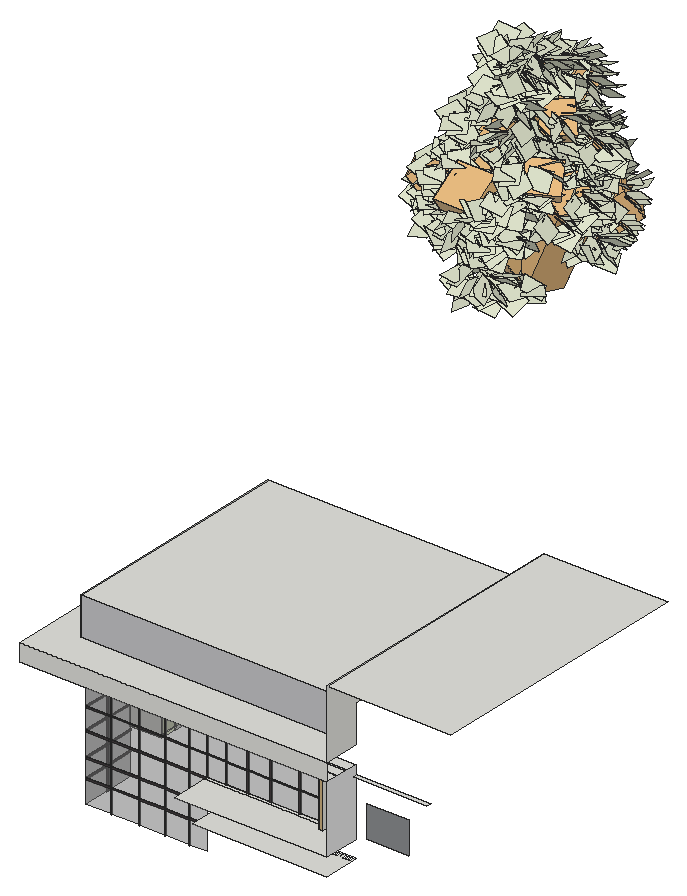
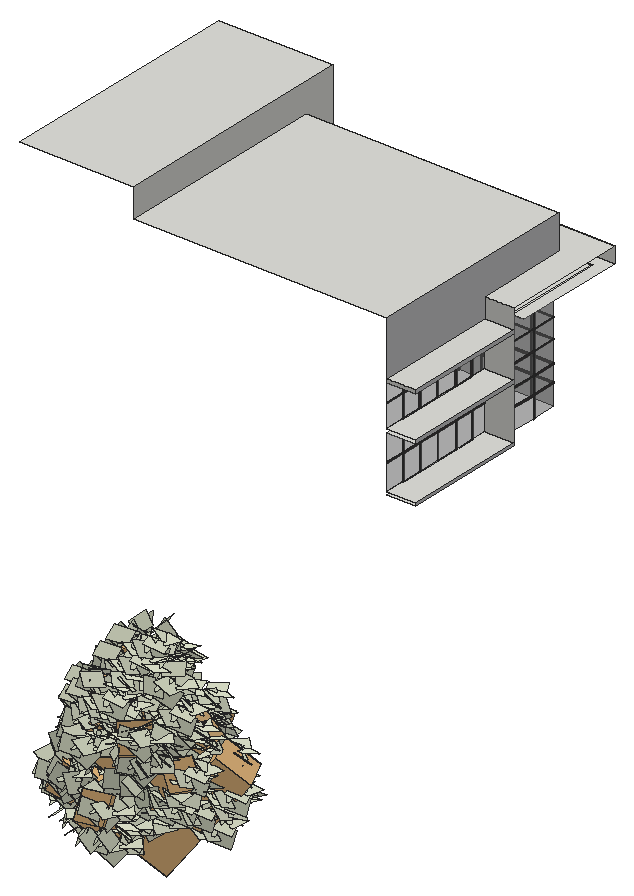
# SketchUp Ruby script. Lengths in inches.
U = 1.inch
M = Sketchup.active_model
def pt(a) = Geom::Point3d.new(a.map { |v| v * U })
def face(e, loops, mat)
  f = e.add_face(loops[0].map { |a| pt(a) })
  loops[1..].each { |l| e.add_face(l.map { |a| pt(a) }).erase! }
  f.material = f.back_material = mat if mat
  f
end
# faces: each face lists its corners as indices into pts; further lists are holes
def faces(e, pts, list, mat = nil) = list.each { |f| face(e, (f[0].is_a?(Array) ? f : [f]).map { |l| l.map { |i| pts[i] } }, mat) }
# xy, xz, yz: faces in a plane at the given z, y or x. An outline is a flat list of corners, or four numbers for a rectangle; further outlines are holes
def ring(l) = l.size == 4 ? [[l[0], l[1]], [l[2], l[1]], [l[2], l[3]], [l[0], l[3]]] : l.each_slice(2).to_a
def flat(e, list, mat, &to3) = list.each { |f| face(e, (f[0].is_a?(Array) ? f : [f]).map { |l| ring(l).map { |u, v| to3.(u, v) } }, mat) }
def xy(e, z, list, mat = nil) = flat(e, list, mat) { |x, y| [x, y, z] }
def xz(e, y, list, mat = nil) = flat(e, list, mat) { |x, z| [x, y, z] }
def yz(e, x, list, mat = nil) = flat(e, list, mat) { |y, z| [x, y, z] }
def lines(e, pts, list) = list.each { |a, b| e.add_line(pt(pts[a]), pt(pts[b])) }
# prism: a flat outline (further loops are holes) pulled along v
def prism(e, loops, v, mat = nil)
  f = face(e, loops, mat); d = Geom::Vector3d.new(v.map { |x| x * U })
  f.pushpull(f.normal.samedirection?(d) ? d.length : -d.length)
end
def box(e, o, s, mat = nil) = prism(e, [[o, [o[0] + s[0], o[1], o[2]], [o[0] + s[0], o[1] + s[1], o[2]], [o[0], o[1] + s[1], o[2]]]], [0, 0, s[2]], mat)
def at(x, y, z, deg = 0) = Geom::Transformation.translation(pt([x, y, z])) * Geom::Transformation.rotation(ORIGIN, Z_AXIS, deg.degrees)
def axes(o, x, y, z) = Geom::Transformation.new([*x, 0, *y, 0, *z, 0, *pt(o).to_a, 1])
def part(name) = M.definitions.add(name)
# library, detail: a bought-in or finely detailed component or shape, given as its bounding box
def library(name, o, s) = part(name).tap { |d| box(d.entities, o, s) }
def detail(e, o, s) = box(e.add_group.entities, o, s)
def put(e, d, t, mat = nil) = e.add_instance(d, t).tap { |i| i.material = mat if mat }
def group(e, t, mat = nil) = e.add_group.tap { |g| g.transformation = t; g.material = mat if mat }.entities
root = M.entities
M.materials.add("Celtis_australis_s cópia1").color = [224, 229, 205]
M.materials.add("Screenshot").color = [140, 142, 145]
M.materials.add("[Asphalt New]").color = [67, 60, 62]
M.materials.add("[Polished Concrete New]").color = [200, 200, 203]
M.materials.add("[Polished Concrete Old]").color = [229, 229, 229]
M.materials.add("[Translucent Glass Gray]").color = [128, 128, 128]
M.materials["[Translucent Glass Gray]"].alpha = 0.5
M.materials.add("[Wood Floor Light]").color = [204, 176, 127]
M.materials.add("bark_cherry").color = [99, 76, 62]
c1 = part("branch2\#1")
p = [[13.74,0.36,0.5],[11.5,11.3125,10.98],[14.125,0.95,0],[14.97,0.95,0.19],[12.12,10.6875,11.67],[15.1,0.36,0.82],
  [11.05,10.4375,11.49],[14.34,0,1.01],[6.08,18.54,23.51],[6.83,18.32,23.89],[6.09,17.93,24.13],[3.27,29.37,34],
  [3.27,29.68,33.56],[3.73,29.59,33.82],[0,43.16,40.74],[0,43.16,40.75],[0.01,43.16,40.75],[5.59,23.2,32.77],
  [4.65,30.48,39.08],[1.92,39.79,43.02],[5.09,28.47,41.41]]
faces(c1.entities,p,[[0,1,2],[2,1,3],[3,4,5],[3,1,4],[6,0,7],[0,6,1],[5,6,7],[6,5,4],
  [6,8,1],[1,9,4],[9,1,8],[8,6,10],[4,10,6],[10,4,9],[10,11,8],[8,12,9],
  [12,8,11],[10,9,11],[13,11,9],[13,9,12],[14,12,11,15],[12,14,16,13],[13,16,15,11]],"bark_cherry")
lines(c1.entities,p,[[17,18],[11,19],[20,17],[17,10]])
c2 = library("branch1\#2",[0,0,0],[33.4,33.29,108.01])
c3 = part("leaf1\#1")
p = [[1.6,6.78,0.04],[-9.34,-4.04,0.02],[2.67,-16.2,2.05],[13.62,-5.38,2.07]]
faces(c3.entities,p,[[0,1,2,3]],"Celtis_australis_s cópia1")
c4 = part("leaf_group1\#1")
put(c4.entities,c3,axes([-0.06,3.68,7.3125],[0.53029,-0.80282,-0.27253],[0.82812,0.42159,0.36943],[-0.18168,-0.42159,0.8884]))
put(c4.entities,c3,axes([6.4375,-3.58,5.23],[1,0,0],[0,0.98927,0.14608],[0,-0.14608,0.98927]))
put(c4.entities,c3,axes([-0.99,3.68,1.22],[0.57591,-0.80282,0.15431],[0.36532,0.42159,0.82994],[-0.73135,-0.42159,0.53609]))
put(c4.entities,c3,axes([18.71,8.59,4.39],[0.33053,0.77491,0.53877],[-0.79988,-0.073,0.5957],[0.50094,-0.62785,0.5957]))
put(c4.entities,c3,axes([13.16,0.76,0.89],[0.89618,0.3501,0.27256],[-0.44248,0.65988,0.60727],[0.03275,-0.66482,0.74628]))
put(c4.entities,c3,axes([4.53,7.98,7.3125],[-0.1927,0.94265,-0.27253],[0.88368,0.28746,0.36943],[-0.42658,0.16964,0.8884]))
put(c4.entities,c3,axes([12.46,21.28,7.16],[0.85019,0.38493,0.35918],[0.30538,-0.91629,0.25914],[-0.42887,0.11063,0.89657]))
put(c4.entities,c3,axes([6.53,15.18,2.59],[0.70711,0.70711,0],[0.5,-0.5,0.70711],[-0.5,0.5,0.70711]))
put(c4.entities,c3,axes([-3.17,8.15,3.46],[-0.03719,0.74973,0.66069],[0.94096,-0.19634,0.27576],[-0.33647,-0.63194,0.69817]))
put(c4.entities,c3,axes([23.03,17.79,4.39],[0.78166,-0.31422,0.53877],[-0.61722,-0.51398,0.5957],[-0.08973,0.79818,0.5957]))
put(c4.entities,c3,axes([14.78,21.52,3.21],[0.67246,-0.04394,0.73882],[-0.28657,-0.93583,0.20517],[-0.6824,0.3497,0.64191]))
put(c4.entities,c3,axes([10.37,-1.8125,9],[0.99279,-0.06448,-0.101],[0.11527,0.74421,0.65792],[0.03275,-0.66482,0.74628]))
put(c4.entities,c3,axes([1.45,16.1875,2.9375],[-0.2106,-0.86579,-0.45394],[0.96054,-0.26957,0.06852],[-0.18168,-0.42159,0.8884]))
c5 = part("branch3")
p = [[6.085,7.082,2.644],[4.083,0.001,0],[4.08,0.002,0.001],[5.841,7.141,2.739],[4.083,0,0.004],[6.032,7.035,2.901],
  [8.234,14.378,3.666],[10.055,21.673,1.937],[8.611,14.241,3.496],[10.247,21.661,2.456],[9.737,21.9,2.346],[9.715,21.803,2.365],
  [12.357,28.999,2.225],[12.894,28.763,2.608],[12.761,28.844,2.204],[10.064,22.087,2.083],[10.362,21.9,2.346],[5.434,16.028,3.111],
  [10.04,22.14,2.516],[12.239,29.014,2.642],[8.553,14.232,3.928],[5.628,15.927,3.273],[5.444,16.098,3.367],[12.571,28.869,2.879],
  [0.628,10.534,6.01],[0.625,10.536,6.008],[0.625,10.537,6.012],[6.135,9.846,4.735],[0.003,10.534,6.01],[0,10.537,6.012],
  [1.761,10.232,4.093],[4.16,5.476,4.049],[3.718,5.459,5.543],[3.205,0.783,1.919]]
faces(c5.entities,p,[[0,1,2,3],[3,2,4,5],[1,0,5,4],[6,7,8],[9,8,7],[7,6,10,11],[12,7,11],[13,7,14],
  [14,7,12],[13,9,7],[15,16,17],[15,17,18],[12,11,19],[20,10,6],[10,20,9,11],[21,17,16],
  [21,16,22],[18,22,16],[9,19,11],[8,9,20],[22,18,17],[9,13,23],[19,9,23],[0,8,5],
  [3,6,0],[8,0,6],[3,5,6],[20,5,8],[20,6,5],[21,24,25,17],[26,22,17,25],[22,26,24,21]],"bark_cherry")
lines(c5.entities,p,[[27,20],[28,29],[17,30],[27,31],[32,27],[5,33]])
c6 = part("branch1\#1")
p = [[23.875,19.65,51.47],[23.47,20.4,51.62],[21.1,21.64,19.5],[21.93,21.1875,19.92],[21.95,22.18,19.69],[26.48,9.62,42.86],
  [30.79,16.22,49.68],[31.01,4.77,55.38],[31.01,0,68.57],[9.91,24.21,59.69],[9.92,24.21,59.7],[24,20.54,51.64],
  [12.85,4.92,53.79],[26.1,8.92,42.74],[31.84,25.13,88.91],[31.84,25.13,106.45],[30.18,33.29,93.95],[30.18,25.42,69.53],
  [0,6.37,81.52],[11.1,10.75,77.87]]
lines(c6.entities,p,[[0,1],[2,3],[3,4],[5,6],[7,8],[9,10],[1,11],[11,0],[12,13],[4,2],[14,15],[16,17],
  [18,19]])
detail(c6.entities,[5.26,2.24,0],[28.14,24.14,108.01])
xy(root,56.77,[[542.91,273.58,570.41,390.8]])
xy(root,59.17,[[542.91,273.58,570.41,390.8]])
xy(root,86.125,[[694.73,152.69,694.73,184.77,755.09,184.77,755.09,179.27,756.79,179.27,756.79,184.77,757.59,184.77,757.59,179.27,759.29,179.27,759.29,184.77,760.09,184.77,760.09,179.27,761.79,179.27,761.79,184.77,762.59,184.77,762.59,179.27,764.29,179.27,764.29,184.77,765.09,184.77,765.09,179.27,766.79,179.27,766.79,184.77,767.59,184.77,767.59,179.27,769.29,179.27,769.29,184.77,770.09,184.77,770.09,179.27,771.79,179.27,771.79,184.77,772.59,184.77,772.59,179.27,774.29,179.27,774.29,184.77,775.09,184.77,775.09,179.27,776.79,179.27,776.79,184.77,777.59,184.77,777.59,179.27,779.29,179.27,779.29,184.77,780.09,184.77,780.09,179.27,781.79,179.27,781.79,184.77,782.59,184.77,782.59,179.27,784.29,179.27,784.29,184.77,785.09,184.77,785.09,179.27,786.79,179.27,786.79,184.77,787.59,184.77,787.59,179.27,789.29,179.27,789.29,184.77,790.09,184.77,790.09,179.27,791.79,179.27,791.79,184.77,792.59,184.77,792.59,179.27,794.29,179.27,794.29,184.77,795.47,184.77,795.47,179.27,797.16,179.27,797.16,184.77,798.34,184.77,798.34,179.27,800.04,179.27,800.04,184.77,801.22,184.77,801.22,179.27,802.91,179.27,802.91,184.77,804.09,184.77,804.09,179.27,805.79,179.27,805.79,184.77,806.97,184.77,806.97,179.27,808.66,179.27,808.66,184.77,809.84,184.77,809.84,179.27,811.54,179.27,811.54,184.77,812.47,184.77,812.47,152.69]])
xy(root,101.125,[[679.09,152.69,812.47,152.69,812.47,184.77,786.97,184.77,786.97,179.89,783.34,179.89,783.34,185.64,679.09,185.64],[679.09,185.64,783.34,188.52]])
xy(root,110.22,[[542.91,273.58,570.41,390.8]])
xy(root,113.5,[[542.91,273.58,570.41,390.8]])
xy(root,143.35,[[565.41,179.89,565.41,237.58,570.41,237.58,570.41,185.64,783.34,185.64,783.34,179.89],[570.41,185.64,570.41,188.45,572.41,185.64],[572.41,185.64,570.41,188.45,570.41,237.58,572.41,237.58,572.41,188.52,783.34,188.52,783.34,185.64]])
xy(root,146.5,[[565.41,179.89,783.34,179.89,783.34,184.77,570.41,184.77,570.41,241.02,565.41,241.02],[783.34,179.89,786.97,184.77]])
xy(root,152.71,[[542.91,273.58,570.41,390.8]])
xy(root,156.52,[[542.91,273.58,570.41,390.8]])
xy(root,160.15,[[542.91,152.69,542.91,261.08,554.03,261.08,554.03,163.32,812.47,163.32,812.47,152.69],[554.03,163.32,554.03,261.08,555.09,261.08,555.09,164.69,812.47,164.69,812.47,163.32],[555.09,164.69,555.09,261.08,559.28,261.08,559.28,173.1,812.47,173.1,812.47,164.69],[559.28,173.1,559.28,261.08,560.36,261.08,560.36,174.73,812.47,174.73,812.47,173.1],[560.36,174.73,560.36,261.08,570.41,261.08,570.41,184.77,812.47,184.77,812.47,174.73]])
xy(root,175.33,[[839.12,148.44,903.81,152.69]])
xy(root,175.35,[[542.91,152.69,812.47,152.69,812.47,184.77,570.41,184.77,570.41,273.58,542.91,273.58]])
xy(root,208.1875,[[570.41,184.77,812.47,390.8]])
xy(root,235.625,[[812.47,152.69,921.28,390.8]])
xz(root,148.44,[[850.82,130.92,887.85,158.83]],"Screenshot")
xz(root,152.69,[[542.91,160.15,812.47,175.35]])
xz(root,179.89,[[783.34,101.125,786.97,146.5],[565.41,143.35,783.34,146.5]],"[Wood Floor Light]")
xz(root,184.77,[[786.97,101.125,812.47,101.125,812.47,160.15,570.41,160.15,570.41,146.5,786.97,146.5]])
xz(root,184.77,[[570.41,175.35,812.47,208.1875]],"[Polished Concrete New]")
xz(root,188.52,[[593.95,42.44,594.71,62.36],[618.47,42.44,619.6,62.36],[641.13,42.44,642.0625,62.36],[662.45,42.44,663.59,62.36],[572.41,62.36,593.95,63.78],
  [593.95,62.36,594.71,63.78],[594.71,62.36,618.47,63.78],[618.47,62.36,619.6,63.78],[619.6,62.36,641.13,63.78],[641.13,62.36,642.0625,63.78],
  [642.0625,62.36,662.45,63.78],[662.45,62.36,663.59,63.78],[663.59,62.36,679.09,63.78],[593.95,63.78,594.71,78.79],[618.47,63.78,619.6,78.79],
  [641.13,63.78,642.0625,78.79],[662.45,63.78,663.59,78.79],[572.41,78.79,593.95,80.28],[593.95,78.79,594.71,80.28],[594.71,78.79,606.59,80.28],
  [606.59,78.79,618.47,80.28],[618.47,78.79,619.6,80.28],[619.6,78.79,641.13,80.28],[641.13,78.79,642.0625,80.28],[642.0625,78.79,662.45,80.28],
  [662.45,78.79,663.59,80.28],[663.59,78.79,679.09,80.28],[593.95,80.28,594.71,99.76],[618.47,80.28,619.6,99.76],[641.13,80.28,642.0625,99.76],
  [662.45,80.28,663.59,99.76],[572.41,99.76,593.95,101.125],[593.95,99.76,594.71,101.125],[594.71,99.76,618.47,101.125],[618.47,99.76,619.6,101.125],
  [619.6,99.76,641.13,101.125],[641.13,99.76,642.0625,101.125],[642.0625,99.76,662.45,101.125],[662.45,99.76,663.59,101.125],[663.59,99.76,679.09,101.125],
  [593.95,101.125,594.71,119.02],[618.47,101.125,619.6,119.02],[641.13,101.125,642.0625,119.02],[662.45,101.125,663.59,119.02],[678.43,101.125,679.09,119.02],
  [695.1,101.125,696.03,119.02],[713.93,101.125,715.23,119.02],[734.02,101.125,735.26,119.02],[759.3,101.125,760.48,119.02],[572.41,119.02,593.95,119.9],
  [593.95,119.02,594.71,119.9],[594.71,119.02,618.47,119.9],[618.47,119.02,619.6,119.9],[619.6,119.02,641.13,119.9],[641.13,119.02,642.0625,119.9],
  [642.0625,119.02,662.45,119.9],[662.45,119.02,663.59,119.9],[663.59,119.02,678.43,119.9],[678.43,119.02,679.09,119.9],[679.09,119.02,695.1,119.9],
  [695.1,119.02,696.03,119.9],[696.03,119.02,713.93,119.9],[713.93,119.02,715.23,119.9],[715.23,119.02,734.02,119.9],[734.02,119.02,735.26,119.9],
  [735.26,119.02,759.3,119.9],[759.3,119.02,760.48,119.9],[760.48,119.02,783.34,119.9],[593.95,119.9,594.71,143.35],[618.47,119.9,619.6,143.35],
  [641.13,119.9,642.0625,143.35],[662.45,119.9,663.59,143.35],[678.43,119.9,679.09,143.35],[695.1,119.9,696.03,143.35],[713.93,119.9,715.23,143.35],
  [734.02,119.9,735.26,143.35],[759.3,119.9,760.48,143.35]],"[Asphalt New]")
xz(root,188.52,[[572.41,42.44,593.95,62.36],[594.71,42.44,618.47,62.36],[619.6,42.44,641.13,62.36],[642.0625,42.44,662.45,62.36],[663.59,42.44,679.09,62.36],
  [572.41,63.78,593.95,78.79],[594.71,63.78,618.47,78.79],[619.6,63.78,641.13,78.79],[642.0625,63.78,662.45,78.79],[663.59,63.78,679.09,78.79],
  [572.41,80.28,593.95,99.76],[594.71,80.28,618.47,99.76],[619.6,80.28,641.13,99.76],[642.0625,80.28,662.45,99.76],[663.59,80.28,679.09,99.76],
  [572.41,101.125,593.95,119.02],[594.71,101.125,618.47,119.02],[619.6,101.125,641.13,119.02],[642.0625,101.125,662.45,119.02],[663.59,101.125,678.43,119.02],
  [679.09,101.125,695.1,119.02],[696.03,101.125,713.93,119.02],[715.23,101.125,734.02,119.02],[735.26,101.125,759.3,119.02],[760.48,101.125,783.34,119.02],
  [572.41,119.9,593.95,143.35],[594.71,119.9,618.47,143.35],[619.6,119.9,641.13,143.35],[642.0625,119.9,662.45,143.35],[663.59,119.9,678.43,143.35],
  [679.09,119.9,695.1,143.35],[696.03,119.9,713.93,143.35],[715.23,119.9,734.02,143.35],[735.26,119.9,759.3,143.35],[760.48,119.9,783.34,143.35]],"[Translucent Glass Gray]")
xz(root,273.58,[[542.91,59.17,570.41,110.22],[542.91,113.5,570.41,152.71],[542.91,156.52,570.41,175.35]])
xz(root,390.8,[[542.91,152.71,570.41,156.52]])
yz(root,542.91,[[273.58,56.77,390.8,59.17],[273.58,110.22,390.8,113.5],[273.58,152.71,390.8,156.52]],"[Polished Concrete New]")
yz(root,570.41,[[288.11,56.77,288.9,59.17],[288.9,56.77,307.55,59.17],[307.55,56.77,308.36,59.17],[308.36,56.77,329.67,59.17],[329.67,56.77,330.36,59.17],
  [330.36,56.77,350.49,59.17],[350.49,56.77,350.93,59.17],[350.93,56.77,370.6875,59.17],[370.6875,56.77,371.49,59.17],[288.11,110.22,288.95,113.5],
  [288.95,110.22,307.55,113.5],[307.55,110.22,308.58,113.5],[308.58,110.22,329.67,113.5],[329.67,110.22,330.24,113.5],[330.24,110.22,350.49,113.5],
  [350.49,110.22,351.51,113.5],[351.51,110.22,370.6875,113.5],[370.6875,110.22,371.56,113.5]])
yz(root,570.41,[[288.11,59.17,288.95,83.29],[307.55,59.17,308.58,83.29],[329.67,59.17,330.24,83.29],[350.49,59.17,351.51,83.29],[370.6875,59.17,371.56,83.29],
  [273.58,83.29,288.11,84.69],[288.11,83.29,288.95,84.69],[288.95,83.29,307.55,84.69],[307.55,83.29,308.58,84.69],[308.58,83.29,329.67,84.69],
  [329.67,83.29,330.24,84.69],[330.24,83.29,350.49,84.69],[350.49,83.29,351.51,84.69],[351.51,83.29,370.6875,84.69],[370.6875,83.29,371.56,84.69],
  [371.56,83.29,390.8,84.69],[288.11,84.69,288.95,110.22],[307.55,84.69,308.58,110.22],[329.67,84.69,330.24,110.22],[350.49,84.69,351.51,110.22],
  [370.6875,84.69,371.56,110.22],[288.11,113.5,289.74,134.54],[307.55,113.5,309.18,134.54],[329.67,113.5,331.31,134.54],[350.49,113.5,352.12,134.54],
  [369.92,113.5,371.56,134.54],[273.58,134.54,288.11,135.8125],[288.11,134.54,289.74,135.8125],[289.74,134.54,307.55,135.8125],[307.55,134.54,309.18,135.8125],
  [309.18,134.54,329.67,135.8125],[329.67,134.54,331.31,135.8125],[331.31,134.54,350.49,135.8125],[350.49,134.54,352.12,135.8125],[352.12,134.54,369.92,135.8125],
  [369.92,134.54,371.56,135.8125],[371.56,134.54,390.8,135.8125],[288.11,135.8125,289.74,152.71],[307.55,135.8125,309.18,152.71],[329.67,135.8125,331.31,152.71],
  [350.49,135.8125,352.12,152.71],[369.92,135.8125,371.56,152.71]],"[Asphalt New]")
yz(root,570.41,[[273.58,156.52,273.58,175.35,184.77,175.35,184.77,208.1875,390.8,208.1875,390.8,156.52]],"[Polished Concrete New]")
yz(root,570.41,[[273.58,59.17,288.11,83.29],[288.95,59.17,307.55,83.29],[308.58,59.17,329.67,83.29],[330.24,59.17,350.49,83.29],[351.51,59.17,370.6875,83.29],
  [371.56,59.17,390.8,83.29],[273.58,84.69,288.11,110.22],[288.95,84.69,307.55,110.22],[308.58,84.69,329.67,110.22],[330.24,84.69,350.49,110.22],
  [351.51,84.69,370.6875,110.22],[371.56,84.69,390.8,110.22],[273.58,113.5,288.11,134.54],[289.74,113.5,307.55,134.54],[309.18,113.5,329.67,134.54],
  [331.31,113.5,350.49,134.54],[352.12,113.5,369.92,134.54],[371.56,113.5,390.8,134.54],[273.58,135.8125,288.11,152.71],[289.74,135.8125,307.55,152.71],
  [309.18,135.8125,329.67,152.71],[331.31,135.8125,350.49,152.71],[352.12,135.8125,369.92,152.71],[371.56,135.8125,390.8,152.71]],"[Translucent Glass Gray]")
yz(root,572.41,[[211.54,42.44,213.05,62.36],[188.52,62.36,210.03,63.78],[210.03,62.36,211.54,63.78],[211.54,62.36,213.05,63.78],[213.05,62.36,237.58,63.78],
  [211.54,63.78,213.05,78.79],[188.52,78.79,210.03,80.28],[210.03,78.79,211.54,80.28],[211.54,78.79,213.05,80.28],[213.05,78.79,237.58,80.28],
  [211.54,80.28,213.05,99.76],[188.52,99.76,210.03,101.125],[210.03,99.76,211.54,101.125],[211.54,99.76,213.05,101.125],[213.05,99.76,237.58,101.125],
  [211.54,101.125,213.05,119.02],[188.52,119.02,210.03,119.9],[210.03,119.02,211.54,119.9],[211.54,119.02,213.05,119.9],[213.05,119.02,237.58,119.9],
  [211.54,119.9,213.05,143.35]],"[Asphalt New]")
yz(root,572.41,[[188.52,42.44,211.54,62.36],[213.05,42.44,237.58,62.36],[188.52,63.78,211.54,78.79],[213.05,63.78,237.58,78.79],[188.52,80.28,211.54,99.76],
  [213.05,80.28,237.58,99.76],[188.52,101.125,211.54,119.02],[213.05,101.125,237.58,119.02],[188.52,119.9,211.54,143.35],[213.05,119.9,237.58,143.35]],"[Translucent Glass Gray]")
yz(root,783.34,[[179.89,101.125,185.64,143.35],[185.64,101.125,188.52,143.35]],"[Wood Floor Light]")
yz(root,786.97,[[179.89,101.125,184.77,146.5]])
yz(root,812.47,[[152.69,175.35,152.69,235.625,390.8,235.625,390.8,208.1875,184.77,208.1875,184.77,175.35]])
yz(root,812.47,[[152.69,101.125,184.77,160.15]],"[Polished Concrete Old]")
p = [[570.41,185.64,143.35],[570.41,182.83,143.35],[679.09,185.64,101.125],[677.34,185.64,101.125],[378.47,918.81,240.05],[378.47,923.31,230.18],
  [377.18,908.11,236.88],[377.18,909.49,238.43],[377.94,918.8,233.18],[377.94,913.86,233.18],[377.94,911.8,230.18],[377.18,912.3,238.43]]
lines(root,p,[[0,1],[2,3],[4,5],[6,7],[8,9],[10,9],[11,7]])
put(root,c1,axes([357.32,925.49,62.65],[0.97196,0.23514,0],[0.21224,-0.87728,-0.43051],[0.10123,-0.41844,0.90259]))
put(root,c2,axes([343.46,938.09,49.8],[0.44254,-0.89649,0.02164],[0.71027,0.36515,0.60182],[-0.54743,-0.25096,0.79834]))
put(root,c4,axes([362.8,866.74,71.15],[0.83641,0.52876,-0.14436],[-0.53435,0.84526,0],[0.12202,0.07714,0.98953]))
put(root,c4,axes([395,880.11,75.61],[0.04316,0.98858,-0.14436],[-0.99905,0.04362,0],[0.0063,0.14422,0.98953]))
put(root,c2,axes([385.75,943.81,60.45],[-0.77824,-0.1312,0.03515],[0.11194,-0.5037,0.59821],[-0.07693,0.59428,0.51479]))
put(root,c2,axes([386.3,900.28,64.22],[0.32556,0.94226,-0.07846],[-0.84329,0.32689,0.42662],[0.35066,-0.05964,0.73884]))
put(root,c2,axes([348.7,909.64,61.74],[1,0,0],[0,0.82413,0.56641],[0,-0.56641,0.82413]))
put(root,c4,axes([356.44,879.22,81.96],[0.59551,-0.79027,-0.14436],[0.79864,0.60182,0],[0.08688,-0.11529,0.98953]))
put(root,c4,axes([337.67,913.31,103.24],[0.74616,0.33065,-0.57786],[-0.40514,0.91425,0],[0.52831,0.23411,0.81614]))
put(root,c4,axes([317.67,880.5,103.24],[0.74616,0.33065,-0.57786],[-0.40514,0.91425,0],[0.52831,0.23411,0.81614]))
put(root,c4,axes([354.2,986.52,90.58],[-0.04316,-0.98858,-0.14436],[0.99905,-0.04362,0],[-0.0063,-0.14422,0.98953]))
put(root,c4,axes([370.95,964.89,90.58],[-0.04316,-0.98858,-0.14436],[0.99905,-0.04362,0],[-0.0063,-0.14422,0.98953]))
put(root,c2,axes([390.1875,925.64,72.79],[-0.55221,0.57381,0.07624],[-0.27657,-0.3541,0.66191],[0.45765,0.38748,0.39851]))
put(root,c4,axes([309.45,913.27,88.26],[0.65426,-0.7553,-0.03839],[0.75585,0.65474,0],[0.02513,-0.02902,0.99926]))
put(root,c4,axes([416.48,953.86,98.46],[-0.05351,0.98808,-0.14436],[-0.99854,-0.05408,0],[-0.00781,0.14414,0.98953]))
put(root,c4,axes([406.3,953.86,98.46],[-0.05351,0.98808,-0.14436],[-0.99854,-0.05408,0],[-0.00781,0.14414,0.98953]))
put(root,c4,axes([436.5,928.93,101.58],[-0.66851,0.72955,-0.14436],[-0.73728,-0.67559,0],[-0.09753,0.10643,0.98953]))
put(root,c4,axes([354.2,974.71,101.83],[-0.04316,-0.98858,-0.14436],[0.99905,-0.04362,0],[-0.0063,-0.14422,0.98953]))
put(root,c4,axes([382.23,975.84,103.96],[0.04316,0.98858,-0.14436],[-0.99905,0.04362,0],[0.0063,0.14422,0.98953]))
put(root,c4,axes([381.85,874.34,106.59],[-0.46214,0.87795,0.12502],[-0.88678,-0.45652,-0.07218],[-0.0063,-0.14422,0.98953]))
put(root,c2,axes([366.74,953.02,90.73],[-0.31066,-0.7342,-0.0666],[0.49665,-0.26184,0.56989],[-0.49034,0.16196,0.50173]))
put(root,c4,axes([408.47,929.43,108.58],[0.66851,-0.72955,-0.14436],[0.73728,0.67559,0],[0.09753,-0.10643,0.98953]))
put(root,c4,axes([372.85,903.47,109.75],[0.98953,0,-0.14436],[0,1,0],[0.14436,0,0.98953]))
put(root,c4,axes([310.81,891.8,110.5],[0.66774,0.73026,-0.14436],[-0.73799,0.67481,0],[0.09741,0.10653,0.98953]))
put(root,c4,axes([364.67,975.84,110.9],[0.04316,0.98858,-0.14436],[-0.99905,0.04362,0],[0.0063,0.14422,0.98953]))
put(root,c4,axes([410.02,969.77,110.96],[-0.04316,-0.98858,-0.14436],[0.99905,-0.04362,0],[-0.0063,-0.14422,0.98953]))
put(root,c4,axes([314.82,929.65,107.82],[0.65426,-0.7553,-0.03839],[0.75585,0.65474,0],[0.02513,-0.02902,0.99926]))
put(root,c4,axes([338.41,945.52,112.88],[0.59551,-0.79027,-0.14436],[0.79864,0.60182,0],[0.08688,-0.11529,0.98953]))
put(root,c4,axes([402.41,977.96,123.8125],[0.04393,-0.98858,-0.14412],[0.83213,-0.04362,0.55286],[-0.55284,-0.14422,0.82071]))
put(root,c4,axes([347.91,874.17,121.06],[0.59551,-0.76679,-0.23959],[0.79864,0.59733,0.07334],[0.08688,-0.23502,0.9681]))
put(root,c4,axes([386.92,865.5,121.06],[0.29786,0.92406,-0.23959],[-0.9435,0.32314,0.07334],[0.14519,0.20421,0.9681]))
put(root,c4,axes([421.42,945.49,115.77],[-0.05351,0.98808,-0.14436],[-0.99854,-0.05408,0],[-0.00781,0.14414,0.98953]))
put(root,c4,axes([321,945.54,116.07],[0.59551,-0.79027,-0.14436],[0.79864,0.60182,0],[0.08688,-0.11529,0.98953]))
put(root,c4,axes([350.31,943.375,124.09],[0.84181,0.51031,0.1759],[-0.46746,0.85217,-0.23515],[-0.2699,0.11572,0.95591]))
put(root,c4,axes([372.85,864.78,118.32],[0.98953,0,-0.14436],[0,1,0],[0.14436,0,0.98953]))
put(root,c4,axes([312.1,886.45,121.19],[0.98953,0,-0.14436],[0,1,0],[0.14436,0,0.98953]))
put(root,c4,axes([294.9,913.8,121.19],[0.62273,-0.76901,-0.14436],[0.77715,0.62932,0],[0.09085,-0.11219,0.98953]))
put(root,c4,axes([347.91,871.52,128.84],[0.59551,-0.78385,0.1759],[0.79864,0.55397,-0.23515],[0.08688,0.28052,0.95591]))
put(root,c4,axes([354.2,996.02,123.21],[-0.04316,-0.98858,-0.14436],[0.99905,-0.04362,0],[-0.0063,-0.14422,0.98953]))
put(root,c2,axes([382.43,912.55,105.76],[-0.7431,0.28874,0.0666],[0.24699,0.5042,0.56989],[-0.1223,-0.41079,0.41644]))
put(root,c4,axes([421.42,909.93,126.77],[-0.05351,0.98808,-0.14436],[-0.99854,-0.05408,0],[-0.00781,0.14414,0.98953]))
put(root,c4,axes([408.24,893.95,126.77],[0.85173,0.50371,-0.14436],[-0.50904,0.86074,0],[0.12425,0.07348,0.98953]))
put(root,c4,axes([410.02,977.96,127.9],[-0.04316,-0.98858,-0.14436],[0.99905,-0.04362,0],[-0.0063,-0.14422,0.98953]))
put(root,c4,axes([312.1,891.76,129.38],[0.98953,0,-0.14436],[0,1,0],[0.14436,0,0.98953]))
put(root,c4,axes([328.77,933.03,131.13],[0.83641,0.52876,-0.14436],[-0.53435,0.84526,0],[0.12202,0.07714,0.98953]))
put(root,c4,axes([347.91,897.3,137.68],[0.59551,-0.76679,-0.23959],[0.79864,0.59733,0.07334],[0.08688,-0.23502,0.9681]))
put(root,c4,axes([372.12,850.6875,138.9],[0.84181,0.51031,0.1759],[-0.46746,0.85217,-0.23515],[-0.2699,0.11572,0.95591]))
put(root,c2,axes([393.51,930.82,112.82],[-0.64428,-0.46954,0.0666],[-0.29101,0.48014,0.56989],[0.27972,-0.32475,0.41644]))
put(root,c4,axes([350.31,943.375,139.53],[0.84181,0.51031,0.1759],[-0.46746,0.85217,-0.23515],[-0.2699,0.11572,0.95591]))
put(root,c4,axes([332.09,931.45,167.99],[0.3711,-0.79027,-0.4876],[0.61978,0.60182,-0.50368],[0.69149,-0.11529,0.71313]))
put(root,c4,axes([314.65,933.03,136.75],[0.83641,0.52876,-0.14436],[-0.53435,0.84526,0],[0.12202,0.07714,0.98953]))
put(root,c4,axes([401.39,912.39,136.9],[-0.04316,-0.98858,-0.14436],[0.99905,-0.04362,0],[-0.0063,-0.14422,0.98953]))
put(root,c4,axes([347.91,894.65,145.46],[0.59551,-0.78385,0.1759],[0.79864,0.55397,-0.23515],[0.08688,0.28052,0.95591]))
put(root,c4,axes([429.42,913.53,139.02],[0.04316,0.98858,-0.14436],[-0.99905,0.04362,0],[0.0063,0.14422,0.98953]))
put(root,c2,axes([360.24,914.88,119.89],[-0.13796,0.78519,0.0666],[0.55922,0.04992,0.56989],[-0.41473,-0.10819,0.41644]))
put(root,c4,axes([372.85,864.78,140.75],[0.98953,0,-0.14436],[0,1,0],[0.14436,0,0.98953]))
put(root,c4,axes([312.1,886.45,140.75],[0.98953,0,-0.14436],[0,1,0],[0.14436,0,0.98953]))
put(root,c4,axes([373.81,928.66,145.77],[-0.04316,-0.98858,-0.14436],[0.99905,-0.04362,0],[-0.0063,-0.14422,0.98953]))
put(root,c4,axes([409.95,933.71,146.02],[-0.04316,-0.98858,-0.14436],[0.99905,-0.04362,0],[-0.0063,-0.14422,0.98953]))
put(root,c4,axes([356.44,889.91,146.71],[0.59551,-0.79027,-0.14436],[0.79864,0.60182,0],[0.08688,-0.11529,0.98953]))
put(root,c2,axes([376.08,956.41,126.99],[0.36963,-0.70636,0.0666],[-0.51774,-0.21719,0.56989],[0.28265,0.17853,0.32482]))
put(root,c4,axes([308.29,945.52,147.57],[0.59551,-0.79027,-0.14436],[0.79864,0.60182,0],[0.08688,-0.11529,0.98953]))
put(root,c4,axes([408.34,925.24,147.98],[0.04316,0.98858,-0.14436],[-0.99905,0.04362,0],[0.0063,0.14422,0.98953]))
put(root,c4,axes([420.08,949.39,148.33],[-0.83641,0.52876,-0.14436],[-0.53435,-0.84526,0],[-0.12202,0.07714,0.98953]))
put(root,c4,axes([327.54,931.45,149.79],[0.59576,-0.79027,-0.14332],[0.79863,0.60182,0.00139],[0.08515,-0.11529,0.98968]))
put(root,c4,axes([392.04,865.03,150.78],[-0.46214,0.87795,0.12502],[-0.88678,-0.45652,-0.07218],[-0.0063,-0.14422,0.98953]))
put(root,c4,axes([341.7,967.77,154.65],[-0.04897,-0.98032,0.19123],[0.95241,0.01183,0.30459],[-0.30086,0.19704,0.93309]))
put(root,c4,axes([396.9375,882.49,152.77],[0.59756,0.78872,-0.14436],[-0.79707,0.60388,0],[0.08717,0.11506,0.98953]))
put(root,c4,axes([346.77,951.97,154.58],[0.04229,0.99083,0.12832],[-0.96813,0.00891,0.25028],[0.24685,-0.13481,0.95963]))
put(root,c4,axes([372.12,885,160.46],[0.84181,0.51031,0.1759],[-0.46746,0.85217,-0.23515],[-0.2699,0.11572,0.95591]))
put(root,c2,axes([373.9,957.65,136.3],[-0.5941,-0.51953,0.03515],[0.35927,-0.37036,0.59821],[-0.29023,0.35871,0.39639]))
put(root,c4,axes([334.78,980.52,192.41],[0.3711,-0.79027,-0.4876],[0.61978,0.60182,-0.50368],[0.69149,-0.11529,0.71313]))
put(root,c4,axes([412.4375,941.24,160.4],[0.59756,0.78872,-0.14436],[-0.79707,0.60388,0],[0.08717,0.11506,0.98953]))
put(root,c4,axes([330.57,979.83,164.78],[-0.04897,-0.98032,0.19123],[0.95241,0.01183,0.30459],[-0.30086,0.19704,0.93309]))
put(root,c4,axes([319.53,915.2,162.88],[0.98953,0,-0.14436],[0,1,0],[0.14436,0,0.98953]))
put(root,c4,axes([351.35,912.59,162.88],[-0.98953,0,-0.14436],[0,-1,0],[-0.14436,0,0.98953]))
put(root,c4,axes([381.89,983.83,163.08],[-0.04316,-0.98858,-0.14436],[0.99905,-0.04362,0],[-0.0063,-0.14422,0.98953]))
put(root,c4,axes([373.35,952.03,162.28],[-0.46214,0.87795,0.12502],[-0.88678,-0.45652,-0.07218],[-0.0063,-0.14422,0.98953]))
put(root,c4,axes([337.41,881.56,164.29],[0.98943,0.01382,-0.14436],[-0.01396,0.9999,0],[0.14434,0.00202,0.98953]))
put(root,c2,axes([379.27,919.63,144.65],[-0.7431,0.28874,0.0666],[0.24699,0.5042,0.56989],[-0.09539,-0.32042,0.32482]))
put(root,c4,axes([382.64,953.65,168.07],[0.97051,-0.19308,-0.14436],[0.19512,0.98078,0],[0.14158,-0.02817,0.98953]))
put(root,c4,axes([382.64,885.96,168.07],[0.97051,-0.19308,-0.14436],[0.19512,0.98078,0],[0.14158,-0.02817,0.98953]))
put(root,c4,axes([358.3,890.05,177.09],[0.98039,-0.08879,0.1759],[0.12944,0.9633,-0.23515],[-0.14857,0.25331,0.95591]))
put(root,c4,axes([394.92,964.77,172.13],[-0.04316,-0.98858,-0.14436],[0.99905,-0.04362,0],[-0.0063,-0.14422,0.98953]))
put(root,c4,axes([319.53,923.39,173.63],[0.98953,0,-0.14436],[0,1,0],[0.14436,0,0.98953]))
put(root,c4,axes([392.1875,929.56,173.71],[0.59756,0.78872,-0.14436],[-0.79707,0.60388,0],[0.08717,0.11506,0.98953]))
put(root,c2,axes([370.875,961.1,172.9],[-0.5154,-0.60822,0.0666],[0.39602,-0.39798,-0.56989],[0.27176,-0.19472,0.32482]))
put(root,c4,axes([393.75,943.54,173.82],[-0.47101,-0.87024,-0.14436],[0.87945,-0.47599,0],[-0.06871,-0.12695,0.98953]))
put(root,c4,axes([350.91,965.53,174.41],[-0.46214,0.87795,0.12502],[-0.88678,-0.45652,-0.07218],[-0.0063,-0.14422,0.98953]))
put(root,c4,axes([350.91,952.03,174.41],[-0.46214,0.87795,0.12502],[-0.88678,-0.45652,-0.07218],[-0.0063,-0.14422,0.98953]))
put(root,c4,axes([345.66,902.45,176.13],[0.59551,-0.79027,-0.14436],[0.79864,0.60182,0],[0.08688,-0.11529,0.98953]))
put(root,c4,axes([382.33,923.26,185.69],[0.59551,-0.79027,-0.14436],[-0.79864,-0.60182,0],[0.08688,-0.11529,0.98953]))
put(root,c4,axes([385.83,923.26,185.69],[0.59551,-0.79027,-0.14436],[-0.79864,-0.60182,0],[0.08688,-0.11529,0.98953]))
put(root,c4,axes([330.33,893.84,186.25],[0.97051,-0.19308,-0.14436],[0.19512,0.98078,0],[0.14158,-0.02817,0.98953]))
put(root,c4,axes([328.23,982.58,187.57],[-0.04316,-0.98858,-0.14436],[0.99905,-0.04362,0],[-0.0063,-0.14422,0.98953]))
put(root,c4,axes([327.54,938.52,189.6],[0.59576,-0.79027,-0.14332],[0.79863,0.60182,0.00139],[0.08515,-0.11529,0.98968]))
put(root,c4,axes([378.35,948.39,190.94],[0.59551,-0.79027,-0.14436],[0.79864,0.60182,0],[0.08688,-0.11529,0.98953]))
put(root,c2,axes([365.53,952.32,171.37],[0.48871,-0.35814,0.05062],[-0.28049,-0.32155,0.43312],[0.17031,0.27706,0.31599]))
put(root,c4,axes([342.71,909.7,191.32],[0.93562,-0.32216,-0.14436],[0.32557,0.94552,0],[0.13649,-0.047,0.98953]))
put(root,c1,axes([365.26,947.05,186.37],[0.29715,-0.71035,0],[-0.64116,-0.2682,-0.33149],[-0.21713,-0.09083,0.49344]))
put(root,c4,axes([361.04,963.2,192.57],[0.59551,-0.79027,-0.14436],[0.79864,0.60182,0],[0.08688,-0.11529,0.98953]))
put(root,c4,axes([365.41,938.39,196],[0.59551,-0.79027,-0.14436],[0.79864,0.60182,0],[0.08688,-0.11529,0.98953]))
put(root,c4,axes([378.35,928.58,196],[0.59551,-0.79027,-0.14436],[0.79864,0.60182,0],[0.08688,-0.11529,0.98953]))
put(root,c4,axes([382.33,923.26,196],[0.59551,-0.79027,-0.14436],[-0.79864,-0.60182,0],[0.08688,-0.11529,0.98953]))
put(root,c4,axes([372.29,971.7,196.57],[0.59551,-0.79027,-0.14436],[0.79864,0.60182,0],[0.08688,-0.11529,0.98953]))
put(root,c4,axes([336.9,938.52,231.68],[0.3711,-0.79027,-0.4876],[0.61978,0.60182,-0.50368],[0.69149,-0.11529,0.71313]))
put(root,c1,axes([358.51,934.3,197.68],[0.74841,0.18106,0],[0.16342,-0.6755,-0.33149],[0.07795,-0.3222,0.69499]))
put(root,c4,axes([361.04,977.08,207.94],[0.59551,-0.79027,-0.14436],[0.79864,0.60182,0],[0.08688,-0.11529,0.98953]))
put(root,c4,axes([372.66,963.2,209.44],[0.59551,-0.79027,-0.14436],[0.79864,0.60182,0],[0.08688,-0.11529,0.98953]))
put(root,c4,axes([356.04,905.39,209.73],[0.59576,-0.79027,-0.14332],[0.79863,0.60182,0.00139],[0.08515,-0.11529,0.98968]))
put(root,c4,axes([335.44,944.32,213.48],[0.18564,-0.97211,-0.14332],[0.98229,0.18738,0.00139],[0.0255,-0.14104,0.98968]))
put(root,c4,axes([361.5,895.81,216.41],[0.9012,0.40902,-0.14332],[-0.4131,0.91068,0.00139],[0.13109,0.05795,0.98968]))
put(root,c4,axes([361.34,956.72,217.44],[0.94927,-0.27938,-0.14436],[0.28234,0.95931,0],[0.13848,-0.04076,0.98953]))
put(root,c1,axes([366.36,945.99,201.16],[0.22289,-0.71035,-0.19651],[-0.70016,-0.2682,0.17535],[0.16345,-0.09083,0.51373]))
put(root,c4,axes([372.98,919.44,220.79],[0.98574,0.08818,-0.14332],[-0.08889,0.99604,0.00139],[0.14287,0.01137,0.98968]))
put(root,c1,axes([379.12,933.6,208.42],[-0.59925,-0.02343,-0.24228],[-0.03641,0.39798,0.05158],[-0.19849,-0.08282,0.49893]))
put(root,c4,axes([360.6,945.2,225.94],[0.59551,-0.79027,-0.14436],[0.79864,0.60182,0],[0.08688,-0.11529,0.98953]))
put(root,c1,axes([366.51,928.44,212.59],[0.39588,0.27856,-0.03174],[0.15584,-0.23409,-0.11069],[0.10636,-0.10805,0.37823]))
put(root,c5,axes([392.22,929.29,215.92],[-0.16853,0.67581,-0.06988],[-0.62427,-0.18244,-0.25885],[-0.26812,0,0.64662]))
put(root,c4,axes([371.125,925.35,224.92],[-0.28104,-0.95381,0.10612],[0.95882,-0.27434,0.07351],[-0.041,0.12241,0.99163]))
put(root,c4,axes([360.6,929.08,233.32],[0.59551,-0.79027,-0.14436],[0.79864,0.60182,0],[0.08688,-0.11529,0.98953]))
put(root,c6,axes([380.92,932.59,213.94],[-0.19674,0.14054,0.03807],[-0.11292,-0.18767,0.10927],[0.06856,0.05241,0.16086]))
put(root,c5,at(361.76,901.88,216.62))
put(root,c5,axes([376.23,932.375,243.27],[-0.72608,-0.15932,-0.23629],[0.2243,0.07943,-0.74282],[0.17579,-0.75941,-0.02812]))
